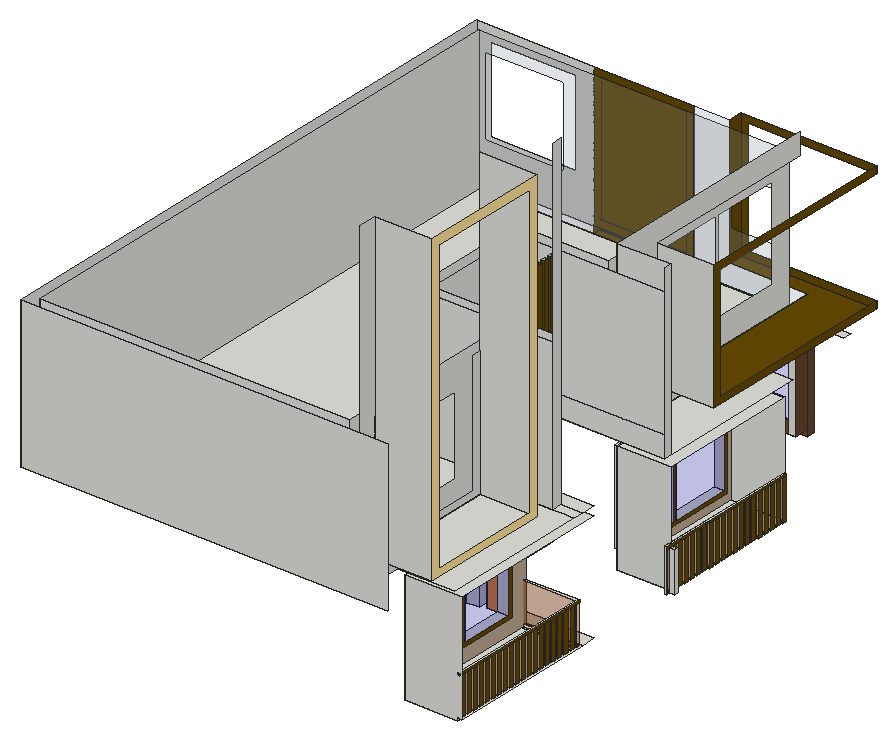
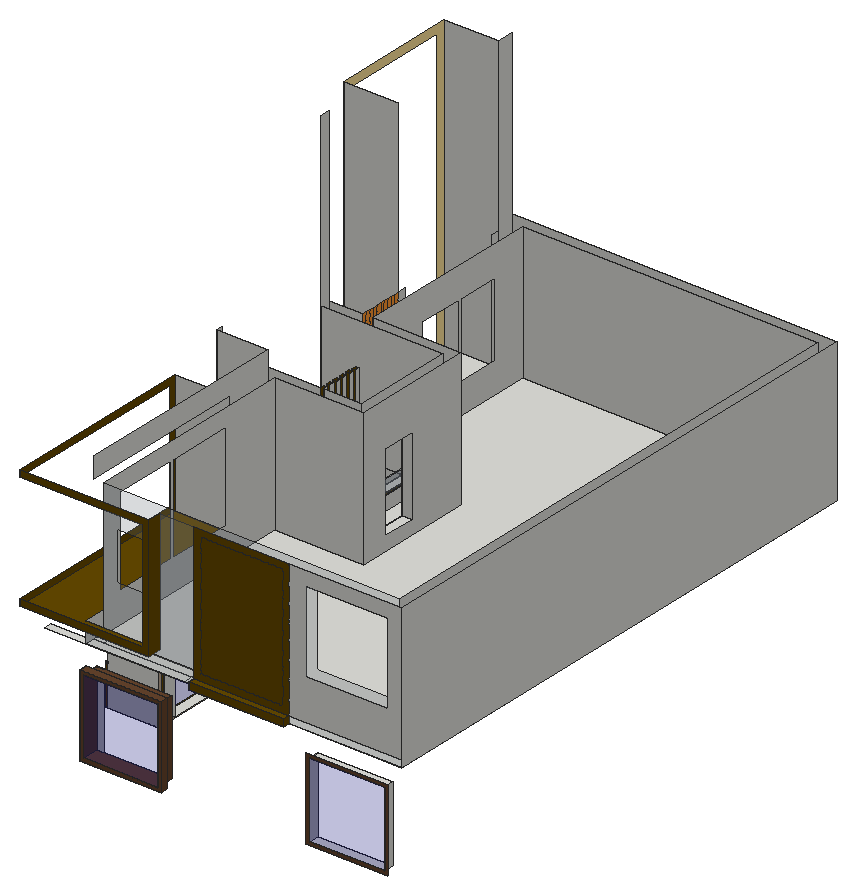
# SketchUp Ruby script. Lengths in inches.
U = 1.inch
M = Sketchup.active_model
def pt(a) = Geom::Point3d.new(a.map { |v| v * U })
def face(e, loops, mat)
  f = e.add_face(loops[0].map { |a| pt(a) })
  loops[1..].each { |l| e.add_face(l.map { |a| pt(a) }).erase! }
  f.material = f.back_material = mat if mat
  f
end
# faces: each face lists its corners as indices into pts; further lists are holes
def faces(e, pts, list, mat = nil) = list.each { |f| face(e, (f[0].is_a?(Array) ? f : [f]).map { |l| l.map { |i| pts[i] } }, mat) }
# xy, xz, yz: faces in a plane at the given z, y or x. An outline is a flat list of corners, or four numbers for a rectangle; further outlines are holes
def ring(l) = l.size == 4 ? [[l[0], l[1]], [l[2], l[1]], [l[2], l[3]], [l[0], l[3]]] : l.each_slice(2).to_a
def flat(e, list, mat, &to3) = list.each { |f| face(e, (f[0].is_a?(Array) ? f : [f]).map { |l| ring(l).map { |u, v| to3.(u, v) } }, mat) }
def xy(e, z, list, mat = nil) = flat(e, list, mat) { |x, y| [x, y, z] }
def xz(e, y, list, mat = nil) = flat(e, list, mat) { |x, z| [x, y, z] }
def yz(e, x, list, mat = nil) = flat(e, list, mat) { |y, z| [x, y, z] }
def lines(e, pts, list) = list.each { |a, b| e.add_line(pt(pts[a]), pt(pts[b])) }
# prism: a flat outline (further loops are holes) pulled along v
def prism(e, loops, v, mat = nil)
  f = face(e, loops, mat); d = Geom::Vector3d.new(v.map { |x| x * U })
  f.pushpull(f.normal.samedirection?(d) ? d.length : -d.length)
end
def box(e, o, s, mat = nil) = prism(e, [[o, [o[0] + s[0], o[1], o[2]], [o[0] + s[0], o[1] + s[1], o[2]], [o[0], o[1] + s[1], o[2]]]], [0, 0, s[2]], mat)
def at(x, y, z, deg = 0) = Geom::Transformation.translation(pt([x, y, z])) * Geom::Transformation.rotation(ORIGIN, Z_AXIS, deg.degrees)
def axes(o, x, y, z) = Geom::Transformation.new([*x, 0, *y, 0, *z, 0, *pt(o).to_a, 1])
def part(name) = M.definitions.add(name)
# library, detail: a bought-in or finely detailed component or shape, given as its bounding box
def library(name, o, s) = part(name).tap { |d| box(d.entities, o, s) }
def detail(e, o, s) = box(e.add_group.entities, o, s)
def put(e, d, t, mat = nil) = e.add_instance(d, t).tap { |i| i.material = mat if mat }
def group(e, t, mat = nil) = e.add_group.tap { |g| g.transformation = t; g.material = mat if mat }.entities
root = M.entities
M.materials.add("C04_Amber_Sunshine").color = [255, 152, 49]
M.materials.add("D02_Buttercup_Glow").color = [255, 229, 155]
M.materials.add("D08_Bronzed_Mustard").color = [102, 74, 0]
M.materials.add("Glass_Basic_01").color = [161, 173, 186]
M.materials["Glass_Basic_01"].alpha = 0.25
M.materials.add("Glass_Sky Reflection_01").color = [130, 55, 3]
M.materials["Glass_Sky Reflection_01"].alpha = 0.25
M.materials.add("Glass_Sky Reflection_1").color = [0, 2, 183]
M.materials["Glass_Sky Reflection_1"].alpha = 0.25
M.materials.add("ThomThom - Complexion1").color = [190, 169, 148]
M.materials.add("Wood_Veneer_15_1K").color = [103, 69, 45]
xy(root,444,[[279,67.85,322.5,190.5],[322.5,67.85,324,67.85,324,192,279,192,279,190.5,322.5,190.5],[324,285,325.5,288.23],[324,288.23,330,291],[279,291,322.5,411],
  [322.5,291,324,411],[324,291.45,325.5,294.68],[324,297.9,325.5,301.125],[324,304.35,325.5,307.58],[324,310.8,325.5,314.03],
  [324,317.25,325.5,320.48],[324,323.7,325.5,326.93],[324,330.15,325.5,333.375],[324,336.6,325.5,339.83],[324,343.05,325.5,346.28],
  [324,349.5,325.5,352.73],[324,355.95,325.5,359.18],[324,362.4,325.5,365.625],[324,368.85,325.5,372.08],[324,375.3,325.5,378.52],
  [324,381.75,325.5,384.98],[324,388.2,325.5,391.42],[324,394.65,325.5,397.875],[324,401.1,325.5,404.32],[324,407.55,325.5,410.77]])
xy(root,445.85,[[324,67.85,327,67.85,327,195,279,195,279,193.5,325.5,193.5,325.5,190.3125,324,190.3125,324,187.125,325.5,187.125,325.5,183.9375,324,183.9375,324,180.75,325.5,180.75,325.5,177.5625,324,177.5625,324,174.375,325.5,174.375,325.5,171.1875,324,171.1875,324,168,325.5,168,325.5,164.8125,324,164.8125,324,161.625,325.5,161.625,325.5,158.4375,324,158.4375,324,155.25,325.5,155.25,325.5,152.0625,324,152.0625,324,148.875,325.5,148.875,325.5,145.6875,324,145.6875,324,142.5,325.5,142.5,325.5,139.3125,324,139.3125,324,136.125,325.5,136.125,325.5,132.9375,324,132.9375,324,129.75,325.5,129.75,325.5,126.5625,324,126.5625,324,123.375,325.5,123.375,325.5,120.1875,324,120.1875,324,117,325.5,117,325.5,113.8125,324,113.8125,324,110.625,325.5,110.625,325.5,107.4375,324,107.4375,324,104.25,325.5,104.25,325.5,101.0625,324,101.0625,324,97.875,325.5,97.875,325.5,94.6875,324,94.6875,324,91.5,325.5,91.5,325.5,88.3125,324,88.3125,324,85.125,325.5,85.125,325.5,81.9375,324,81.9375,324,78.75,325.5,78.75,325.5,75.5625,324,75.5625,324,72.375,325.5,72.375,325.5,69.1875,324,69.1875],[246,195,327,207.17]])
xy(root,450,[[228,195,229.5,285]])
xy(root,453,[[270,300,279,350.5],[270,352.5,279,405]])
xy(root,456,[[207,492,279,498]],"Wood_Veneer_15_1K")
xy(root,459,[[270,81,279,129],[270,131,279,177],[15,483,81,492]])
xy(root,459,[[210,483,276,498]],"Wood_Veneer_15_1K")
xy(root,478,[[325.5,288.23,330,291]])
xy(root,478,[[324,67.85,325.5,69.1875],[324,72.375,325.5,75.5625],[324,78.75,325.5,81.9375],[324,85.125,325.5,88.3125],[324,91.5,325.5,94.6875],
  [324,97.875,325.5,101.0625],[324,104.25,325.5,107.4375],[324,110.625,325.5,113.8125],[324,117,325.5,120.1875],[324,123.375,325.5,126.5625],
  [324,129.75,325.5,132.9375],[324,136.125,325.5,139.3125],[324,142.5,325.5,145.6875],[324,148.875,325.5,152.0625],[324,155.25,325.5,158.4375],
  [324,161.625,325.5,164.8125],[324,168,325.5,171.1875],[324,174.375,325.5,177.5625],[324,180.75,325.5,183.9375],[324,187.125,325.5,190.3125],
  [324,288.23,325.5,291],[324,291,325.5,291.45],[324,294.68,325.5,297.9],[324,301.125,325.5,304.35],[324,307.58,325.5,310.8],
  [324,314.03,325.5,317.25],[324,320.48,325.5,323.7],[324,326.92,325.5,330.15],[324,333.375,325.5,336.6],[324,339.82,325.5,343.05],
  [325.5,346.27,324,346.28,324,349.5,325.5,349.5],[324,352.72,325.5,355.95],[324,359.17,325.5,362.4],[324,365.625,325.5,368.85],[324,372.07,325.5,375.3],
  [324,378.52,325.5,381.75],[324,384.97,325.5,388.2],[324,391.42,325.5,394.65],[324,397.875,325.5,401.1],[324,404.32,325.5,407.55],
  [324,410.77,325.5,411]],"Glass_Sky Reflection_01")
xy(root,480,[[324,67.85,325.5,67.85,325.5,193.5,279,193.5,279,192,324,192],[324,285,325.5,411]])
xy(root,507,[[192,240,201,270]])
xy(root,525,[[270,81,279,129],[270,131,279,177],[15,483,81,492]])
xy(root,525,[[210,483,276,498]],"Wood_Veneer_15_1K")
xy(root,528,[[207,492,279,498]],"Wood_Veneer_15_1K")
xy(root,531,[[270,300,279,350.5],[270,352.5,279,405]])
xy(root,537,[[279,291,324,411]])
xy(root,538.15,[[279,67.85,279,195,246,195,246,207.17,327,207.17,327,67.85]])
xy(root,546,[[0,21,9,483],[9,21,9,483,192,483,192,186,270,186,270,21],[270,21,279,21,279,186,309,186,309,195,270,195],[279,60,327,186],[192,186,270,186,270,195,201,195,201,285,324,285,324,291,279,291,279,294,192,294],
  [309,186,327,195],[201,195,201,285,237,285,237,237,234,237,234,233.5,237,233.5,237,230,234,230,234,226.5,237,226.5,237,223,234,223,234,219.5,237,219.5,237,216,234,216,234,212.5,237,212.5,237,209,234,209,234,205.5,237,205.5,237,202,234,202,234,198.5,237,198.5,237,195],[240,195,327,207.17],[279,291,324,420],[192,294,270,483],
  [270,294,279,483],[0,483,192,492],[192,483,279,492],[279,484.8,315,492]])
xy(root,546,[[99,492,183,498]],"D08_Bronzed_Mustard")
xy(root,552,[[9,21,270,21,270,186,192,186,192,294,270,294,270,483,9,483],[201,195,226.5,285]])
xy(root,552,[[99,492,183,498]],"D08_Bronzed_Mustard")
xy(root,564,[[279,36,327,147],[226.5,195,228,285],[229.5,195,237,195,237,246.5,234,246.5,234,285,229.5,285],[192,240,201,270],[234,250,237,253.5],
  [234,257,237,260.5],[234,264,237,267.5],[234,271,237,274.5],[234,278,237,281.5]])
xy(root,564,[[279,333,279,492,213,492,213,504,327,504,327,333]],"D08_Bronzed_Mustard")
xz(root,12,[[0,546,309,672]])
xz(root,21,[[9,552,270,672]])
xz(root,36,[[279,564,327,822]])
xz(root,67.85,[[[279,444,279,538.15,327,538.15,327,445.85,324,445.85,324,444],[324,478,325.5,480]]])
xz(root,69.1875,[[324,445.85,325.5,478]],"Glass_Sky Reflection_01")
xz(root,72.375,[[324,445.85,325.5,478]],"Glass_Sky Reflection_01")
xz(root,75.5625,[[324,445.85,325.5,478]],"Glass_Sky Reflection_01")
xz(root,78.75,[[324,445.85,325.5,478]],"Glass_Sky Reflection_01")
xz(root,81,[[270,459,279,525]])
xz(root,81.9375,[[324,445.85,325.5,478]],"Glass_Sky Reflection_01")
xz(root,85.125,[[324,445.85,325.5,478]],"Glass_Sky Reflection_01")
xz(root,88.3125,[[324,445.85,325.5,478]],"Glass_Sky Reflection_01")
xz(root,91.5,[[324,445.85,325.5,478]],"Glass_Sky Reflection_01")
xz(root,94.6875,[[324,445.85,325.5,478]],"Glass_Sky Reflection_01")
xz(root,97.875,[[324,445.85,325.5,478]],"Glass_Sky Reflection_01")
xz(root,101.0625,[[324,445.85,325.5,478]],"Glass_Sky Reflection_01")
xz(root,104.25,[[324,445.85,325.5,478]],"Glass_Sky Reflection_01")
xz(root,107.4375,[[324,445.85,325.5,478]],"Glass_Sky Reflection_01")
xz(root,110.625,[[324,445.85,325.5,478]],"Glass_Sky Reflection_01")
xz(root,113.8125,[[324,445.85,325.5,478]],"Glass_Sky Reflection_01")
xz(root,117,[[324,445.85,325.5,478]],"Glass_Sky Reflection_01")
xz(root,120.1875,[[324,445.85,325.5,478]],"Glass_Sky Reflection_01")
xz(root,123.375,[[324,445.85,325.5,478]],"Glass_Sky Reflection_01")
xz(root,126.5625,[[324,445.85,325.5,478]],"Glass_Sky Reflection_01")
xz(root,129,[[270,459,279,525]])
xz(root,129.75,[[324,445.85,325.5,478]],"Glass_Sky Reflection_01")
xz(root,131,[[270,459,279,525]])
xz(root,132.9375,[[324,445.85,325.5,478]],"Glass_Sky Reflection_01")
xz(root,136.125,[[324,445.85,325.5,478]],"Glass_Sky Reflection_01")
xz(root,139.3125,[[324,445.85,325.5,478]],"Glass_Sky Reflection_01")
xz(root,142.5,[[324,445.85,325.5,478]],"Glass_Sky Reflection_01")
xz(root,145.6875,[[324,445.85,325.5,478]],"Glass_Sky Reflection_01")
xz(root,147,[[279,564,327,822]])
xz(root,148.875,[[324,445.85,325.5,478]],"Glass_Sky Reflection_01")
xz(root,152.0625,[[324,445.85,325.5,478]],"Glass_Sky Reflection_01")
xz(root,155.25,[[324,445.85,325.5,478]],"Glass_Sky Reflection_01")
xz(root,158.4375,[[324,445.85,325.5,478]],"Glass_Sky Reflection_01")
xz(root,161.625,[[324,445.85,325.5,478]],"Glass_Sky Reflection_01")
xz(root,164.8125,[[324,445.85,325.5,478]],"Glass_Sky Reflection_01")
xz(root,168,[[324,445.85,325.5,478]],"Glass_Sky Reflection_01")
xz(root,171.1875,[[324,445.85,325.5,478]],"Glass_Sky Reflection_01")
xz(root,174.375,[[324,445.85,325.5,478]],"Glass_Sky Reflection_01")
xz(root,177,[[270,459,279,525]])
xz(root,177.5625,[[324,445.85,325.5,478]],"Glass_Sky Reflection_01")
xz(root,180.75,[[324,445.85,325.5,478]],"Glass_Sky Reflection_01")
xz(root,183.9375,[[324,445.85,325.5,478]],"Glass_Sky Reflection_01")
xz(root,186,[[279,546,309,672],[192,552,270,672]])
xz(root,187.125,[[324,445.85,325.5,478]],"Glass_Sky Reflection_01")
xz(root,190.3125,[[324,445.85,325.5,478]],"Glass_Sky Reflection_01")
xz(root,192,[[279,444,324,480]],"Glass_Sky Reflection_01")
xz(root,193.5,[[279,445.85,325.5,480]],"Glass_Sky Reflection_01")
xz(root,195,[[201,444,201,540,240,540,240,444,229.5,444,229.5,450,228,450,228,444],[201,540,240,546],[237,546,309,564],[201,552,226.5,564],[201,564,201,672,309,672,309,564,229.5,564,229.5,576,228,576,228,564]])
xz(root,195,[[246,445.85,279,538.15]],"C04_Amber_Sunshine")
xz(root,240,[[192,564,201,633]])
xz(root,246.5,[[234,564,237,672]],"D08_Bronzed_Mustard")
xz(root,250,[[234,564,237,672]],"D08_Bronzed_Mustard")
xz(root,253.5,[[234,564,237,672]],"D08_Bronzed_Mustard")
xz(root,257,[[234,564,237,672]],"D08_Bronzed_Mustard")
xz(root,260.5,[[234,564,237,672]],"D08_Bronzed_Mustard")
xz(root,264,[[234,564,237,672]],"D08_Bronzed_Mustard")
xz(root,267.5,[[234,564,237,672]],"D08_Bronzed_Mustard")
xz(root,270,[[192,564,201,633]])
xz(root,271,[[234,564,237,672]],"D08_Bronzed_Mustard")
xz(root,274.5,[[234,564,237,672]],"D08_Bronzed_Mustard")
xz(root,278,[[234,564,237,672]],"D08_Bronzed_Mustard")
xz(root,281.5,[[234,564,237,672]],"D08_Bronzed_Mustard")
xz(root,285,[[324,444,325.5,480],[237,546,324,564],[201,552,226.5,564],[201,564,228,564,228,576,229.5,576,229.5,564,234,564,234,672,201,672],[237,564,324,672]])
xz(root,288.23,[[325.5,444,330,478]])
xz(root,288.23,[[324,444,325.5,478]],"Glass_Sky Reflection_01")
xz(root,291,[[279,444,279,537,324,537,324,478,330,478,330,444],[279,546,324,690]])
xz(root,291.45,[[324,444,325.5,478]],"Glass_Sky Reflection_01")
xz(root,294,[[192,552,270,672]])
xz(root,294.68,[[324,444,325.5,478]],"Glass_Sky Reflection_01")
xz(root,297.9,[[324,444,325.5,478]],"Glass_Sky Reflection_01")
xz(root,300,[[270,453,279,531]])
xz(root,301.125,[[324,444,325.5,478]],"Glass_Sky Reflection_01")
xz(root,304.35,[[324,444,325.5,478]],"Glass_Sky Reflection_01")
xz(root,307.58,[[324,444,325.5,478]],"Glass_Sky Reflection_01")
xz(root,310.8,[[324,444,325.5,478]],"Glass_Sky Reflection_01")
xz(root,314.03,[[324,444,325.5,478]],"Glass_Sky Reflection_01")
xz(root,317.25,[[324,444,325.5,478]],"Glass_Sky Reflection_01")
xz(root,320.48,[[324,444,325.5,478]],"Glass_Sky Reflection_01")
xz(root,323.7,[[324,444,325.5,478]],"Glass_Sky Reflection_01")
xz(root,330.15,[[324,444,325.5,478]],"Glass_Sky Reflection_01")
xz(root,333,[[279,564,327,672]])
xz(root,333.375,[[324,444,325.5,478]],"Glass_Sky Reflection_01")
xz(root,336.6,[[324,444,325.5,478]],"Glass_Sky Reflection_01")
xz(root,343.05,[[324,444,325.5,478]],"Glass_Sky Reflection_01")
xz(root,349.5,[[324,444,325.5,478]],"Glass_Sky Reflection_01")
xz(root,350.5,[[270,453,279,531]])
xz(root,352.5,[[270,453,279,531]])
xz(root,355.95,[[324,444,325.5,478]],"Glass_Sky Reflection_01")
xz(root,362.4,[[324,444,325.5,478]],"Glass_Sky Reflection_01")
xz(root,365.625,[[324,444,325.5,478]],"Glass_Sky Reflection_01")
xz(root,368.85,[[324,444,325.5,478]],"Glass_Sky Reflection_01")
xz(root,375.3,[[324,444,325.5,478]],"Glass_Sky Reflection_01")
xz(root,378.52,[[324,444,325.5,478]],"Glass_Sky Reflection_01")
xz(root,381.75,[[324,444,325.5,478]],"Glass_Sky Reflection_01")
xz(root,388.2,[[324,444,325.5,478]],"Glass_Sky Reflection_01")
xz(root,391.42,[[324,444,325.5,478]],"Glass_Sky Reflection_01")
xz(root,394.65,[[324,444,325.5,478]],"Glass_Sky Reflection_01")
xz(root,397.875,[[324,444,325.5,478]],"Glass_Sky Reflection_01")
xz(root,401.1,[[324,444,325.5,478]],"Glass_Sky Reflection_01")
xz(root,404.32,[[324,444,325.5,478]],"Glass_Sky Reflection_01")
xz(root,405,[[270,453,279,531]])
xz(root,407.55,[[324,444,325.5,478]],"Glass_Sky Reflection_01")
xz(root,410.77,[[324,444,325.5,478]],"Glass_Sky Reflection_01")
xz(root,411,[[279,444,324,537],[324,478,325.5,480]])
xz(root,483,[[270,459,276,525]])
xz(root,483,[[[9,552,270,672],[15,591,81,657],[222,597,258,639]]],"Glass_Basic_01")
xz(root,492,[[[0,552,99,672],[12,588,84,660]]])
xz(root,492,[[[99,552,183,672],[105,558,177,666]],[105,558,177,666]],"D08_Bronzed_Mustard")
xz(root,492,[[0,546,99,552],[183,546,183,672,213,672,213,564,279,564,279,546]],"Glass_Basic_01")
xz(root,492,[[15,459,81,525]],"Glass_Sky Reflection_1")
xz(root,492,[[[12,456,84,528],[15,459,81,525]]],"Wood_Veneer_15_1K")
xz(root,498,[[99,546,183,552]],"D08_Bronzed_Mustard")
xz(root,498,[[210,459,276,525]],"Glass_Sky Reflection_1")
xz(root,498,[[[207,456,279,528],[210,459,276,525]]],"Wood_Veneer_15_1K")
xz(root,504,[[213,564,213,672,327,672,327,666,219,666,219,570,327,570,327,564]],"D08_Bronzed_Mustard")
yz(root,0,[[12,546,492,672]])
yz(root,9,[[21,552,483,672]])
yz(root,15,[[483,459,492,525]])
yz(root,81,[[483,459,492,525]])
yz(root,99,[[492,546,498,552]],"D08_Bronzed_Mustard")
yz(root,183,[[492,546,498,552]],"D08_Bronzed_Mustard")
yz(root,192,[[[186,552,294,672],[240,564,270,633]]])
yz(root,201,[[195,552,237,564],[237,552,273,552,273,564,270,564,270,555,240,555,240,564,237,564],[273,552,285,564],[240,555,270,564],[195,564,237,564,237,636,273,636,273,564,285,564,285,672,195,672]])
yz(root,201,[[237,564,240,564,240,633,270,633,270,564,273,564,273,636,237,636]],"D08_Bronzed_Mustard")
yz(root,207,[[492,456,498,528]],"Wood_Veneer_15_1K")
yz(root,210,[[483,459,498,525]],"Wood_Veneer_15_1K")
yz(root,213,[[492,564,504,672]],"D08_Bronzed_Mustard")
yz(root,226.5,[[195,552,285,564]])
yz(root,228,[[195,564,285,576]],"Glass_Basic_01")
yz(root,229.5,[[195,564,285,576]],"Glass_Basic_01")
yz(root,234,[[246.5,564,250,672],[253.5,564,257,672],[260.5,564,264,672],[267.5,564,271,672],[274.5,564,278,672],
  [281.5,564,285,672]])
yz(root,237,[[195,546,246.5,564],[246.5,546,250,672],[250,546,253.5,564],[253.5,546,257,672],[257,546,260.5,564],
  [260.5,546,264,672],[264,546,267.5,564],[267.5,546,271,672],[271,546,274.5,564],[274.5,546,278,672],
  [278,546,281.5,564],[281.5,546,285,672]],"D08_Bronzed_Mustard")
yz(root,240,[[195,444,207.17,540],[195,540,207.17,546]])
yz(root,246,[[195,445.85,207.17,538.15]])
yz(root,270,[[[21,552,186,672],[91.5,579,132,645],[51,579,89.5,645]],[[294,552,483,672],[348,579,406.5,657],[408.5,579,465,657]]])
yz(root,276,[[483,459,498,525]],"Wood_Veneer_15_1K")
yz(root,279,[[21,546,186,546,186,564,36,564,36,822,21,822],[291,546,492,546,492,564,333,564,333,672,483,672,483,690,291,690],[36,564,147,564,147,672,139.15,672,139.15,570,43.85,570,43.85,672,36,672]])
yz(root,279,[[147,564,150.9,672],[150.9,564,154.8,672],[154.8,564,158.7,672],[158.7,564,162.6,672],[162.6,564,166.5,672],
  [166.5,564,170.4,672],[170.4,564,174.3,672],[174.3,564,178.2,672],[178.2,564,182.1,672],[182.1,564,186,672]],"C04_Amber_Sunshine")
yz(root,279,[[[297,450,408,534],[300,453,300,531,350.5,531,350.5,453,352.5,453,352.5,531,405,531,405,453]],[[78,456,180,528],[81,459,81,525,129,525,129,459,131,459,131,525,177,525,177,459]]],"D08_Bronzed_Mustard")
yz(root,279,[[300,453,350.5,531],[352.5,453,405,531],[81,459,129,525],[131,459,177,525]],"Glass_Sky Reflection_1")
yz(root,279,[[[67.85,444,192,444,192,480,193.5,480,193.5,445.85,195,445.85,195,538.15,67.85,538.15],[78,456,180,528]],[[291,444,411,537],[297,450,408,534]]],"ThomThom - Complexion1")
yz(root,279,[[492,456,498,528]],"Wood_Veneer_15_1K")
yz(root,309,[[186,546,195,822]])
yz(root,324,[[67.85,444,69.1875,445.85],[72.375,444,75.5625,445.85],[78.75,444,81.9375,445.85],[85.125,444,88.3125,445.85],[91.5,444,94.6875,445.85],
  [97.875,444,101.0625,445.85],[104.25,444,107.4375,445.85],[110.625,444,113.8125,445.85],[117,444,120.1875,445.85],[123.375,444,126.5625,445.85],
  [129.75,444,132.9375,445.85],[136.125,444,139.3125,445.85],[142.5,444,145.6875,445.85],[148.875,444,152.0625,445.85],[155.25,444,158.4375,445.85],
  [161.625,444,164.8125,445.85],[168,444,171.1875,445.85],[174.375,444,177.5625,445.85],[180.75,444,183.9375,445.85],[187.125,444,190.3125,445.85],
  [285,546,291,690]])
yz(root,324,[[69.1875,444,69.1875,478,67.85,478,67.85,480,192,480,192,444,190.3125,444,190.3125,478,187.125,478,187.125,444,183.9375,444,183.9375,478,180.75,478,180.75,444,177.5625,444,177.5625,478,174.375,478,174.375,444,171.1875,444,171.1875,478,168,478,168,444,164.8125,444,164.8125,478,161.625,478,161.625,444,158.4375,444,158.4375,478,155.25,478,155.25,444,152.0625,444,152.0625,478,148.875,478,148.875,444,145.6875,444,145.6875,478,142.5,478,142.5,444,139.3125,444,139.3125,478,136.125,478,136.125,444,132.9375,444,132.9375,478,129.75,478,129.75,444,126.5625,444,126.5625,478,123.375,478,123.375,444,120.1875,444,120.1875,478,117,478,117,444,113.8125,444,113.8125,478,110.625,478,110.625,444,107.4375,444,107.4375,478,104.25,478,104.25,444,101.0625,444,101.0625,478,97.875,478,97.875,444,94.6875,444,94.6875,478,91.5,478,91.5,444,88.3125,444,88.3125,478,85.125,478,85.125,444,81.9375,444,81.9375,478,78.75,478,78.75,444,75.5625,444,75.5625,478,72.375,478,72.375,444],[285,444,285,480,291,480,291,478,288.23,478,288.23,444],[291.45,444,291.45,478,291,478,291,480,411,480,411,478,410.77,478,410.77,444,407.55,444,407.55,478,404.32,478,404.32,444,401.1,444,401.1,478,397.875,478,397.875,444,394.65,444,394.65,478,391.42,478,391.42,444,388.2,444,388.2,478,384.97,478,384.98,444,381.75,444,381.75,478,378.52,478,378.52,444,375.3,444,375.3,478,372.07,478,372.08,444,368.85,444,368.85,478,365.625,478,365.625,444,362.4,444,362.4,478,359.17,478,359.18,444,355.95,444,355.95,478,352.72,478,352.73,444,349.5,444,349.5,478,346.28,478,346.28,444,343.05,444,343.05,478,339.82,478,339.83,444,336.6,444,336.6,478,333.375,478,333.375,444,330.15,444,330.15,478,326.92,478,326.93,444,323.7,444,323.7,478,320.48,478,320.48,444,317.25,444,317.25,478,314.03,478,314.03,444,310.8,444,310.8,478,307.58,478,307.58,444,304.35,444,304.35,478,301.125,478,301.125,444,297.9,444,297.9,478,294.68,478,294.68,444]],"Glass_Sky Reflection_01")
yz(root,325.5,[[291.45,444,294.68,478],[297.9,444,301.125,478],[304.35,444,307.58,478],[310.8,444,314.03,478],[317.25,444,320.48,478],
  [323.7,444,326.93,444,326.92,478,323.7,478],[330.15,444,333.375,478],[336.6,444,339.83,444,339.82,478,336.6,478],[343.05,444,346.28,444,346.27,478,343.05,478],[349.5,444,352.73,444,352.72,478,349.5,478],
  [355.95,444,359.18,444,359.17,478,355.95,478],[362.4,444,365.625,478],[368.85,444,372.08,444,372.07,478,368.85,478],[375.3,444,378.52,478],[381.75,444,384.98,444,384.97,478,381.75,478],
  [388.2,444,391.42,478],[394.65,444,397.875,478],[401.1,444,404.32,478],[407.55,444,410.77,478],[69.1875,445.85,72.375,478],
  [75.5625,445.85,78.75,478],[81.9375,445.85,85.125,478],[88.3125,445.85,91.5,478],[94.6875,445.85,97.875,478],[101.0625,445.85,104.25,478],
  [107.4375,445.85,110.625,478],[113.8125,445.85,117,478],[120.1875,445.85,123.375,478],[126.5625,445.85,129.75,478],[132.9375,445.85,136.125,478],
  [139.3125,445.85,142.5,478],[145.6875,445.85,148.875,478],[152.0625,445.85,155.25,478],[158.4375,445.85,161.625,478],[164.8125,445.85,168,478],
  [171.1875,445.85,174.375,478],[177.5625,445.85,180.75,478],[183.9375,445.85,187.125,478],[67.85,478,193.5,480],[285,478,326.92,480],
  [326.92,478,330.15,480],[330.15,478,411,480]],"D08_Bronzed_Mustard")
yz(root,325.5,[[285,444,288.23,478],[190.3125,445.85,193.5,478]],"Glass_Sky Reflection_01")
yz(root,327,[[[36,564,147,822],[43.85,570,139.15,814.15]]],"D02_Buttercup_Glow")
yz(root,327,[[333,564,504,564,504,570,339,570,339,666,504,666,504,672,333,672]],"D08_Bronzed_Mustard")
yz(root,330,[[288.23,444,291,478]])
p = [[325.5,326.92,478],[325.5,326.93,444],[324,326.93,444],[324,326.92,478],[325.5,339.82,478],[325.5,339.83,444],
  [324,339.83,444],[324,339.82,478],[325.5,346.27,478],[325.5,346.28,444],[324,346.28,444],[324,346.28,478],
  [325.5,352.72,478],[325.5,352.73,444],[324,352.73,444],[324,352.72,478],[325.5,359.17,478],[325.5,359.18,444],
  [324,359.18,444],[324,359.17,478],[325.5,372.07,478],[325.5,372.08,444],[324,372.08,444],[324,372.07,478],
  [325.5,384.97,478],[325.5,384.98,444],[324,384.98,444],[324,384.97,478]]
faces(root,p,[[0,1,2,3],[4,5,6,7],[8,9,10,11],[12,13,14,15],[16,17,18,19],[20,21,22,23],[24,25,26,27]],"Glass_Sky Reflection_01")
